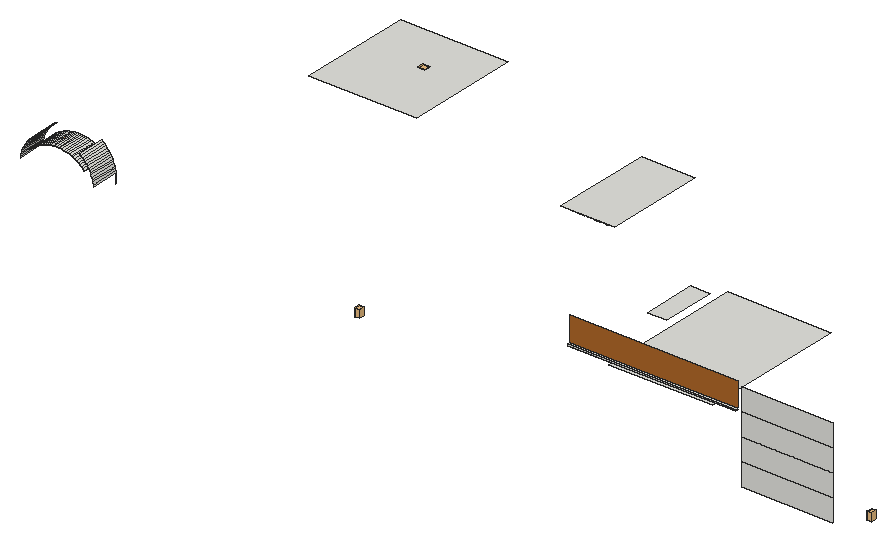
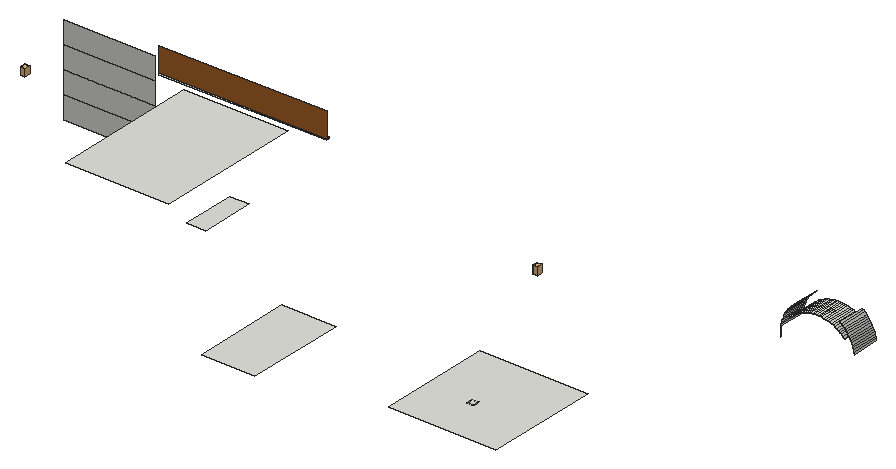
# SketchUp Ruby script. Lengths in inches.
U = 1.inch
M = Sketchup.active_model
def pt(a) = Geom::Point3d.new(a.map { |v| v * U })
def face(e, loops, mat)
  f = e.add_face(loops[0].map { |a| pt(a) })
  loops[1..].each { |l| e.add_face(l.map { |a| pt(a) }).erase! }
  f.material = f.back_material = mat if mat
  f
end
# faces: each face lists its corners as indices into pts; further lists are holes
def faces(e, pts, list, mat = nil) = list.each { |f| face(e, (f[0].is_a?(Array) ? f : [f]).map { |l| l.map { |i| pts[i] } }, mat) }
# xy, xz, yz: faces in a plane at the given z, y or x. An outline is a flat list of corners, or four numbers for a rectangle; further outlines are holes
def ring(l) = l.size == 4 ? [[l[0], l[1]], [l[2], l[1]], [l[2], l[3]], [l[0], l[3]]] : l.each_slice(2).to_a
def flat(e, list, mat, &to3) = list.each { |f| face(e, (f[0].is_a?(Array) ? f : [f]).map { |l| ring(l).map { |u, v| to3.(u, v) } }, mat) }
def xy(e, z, list, mat = nil) = flat(e, list, mat) { |x, y| [x, y, z] }
def xz(e, y, list, mat = nil) = flat(e, list, mat) { |x, z| [x, y, z] }
def yz(e, x, list, mat = nil) = flat(e, list, mat) { |y, z| [x, y, z] }
def lines(e, pts, list) = list.each { |a, b| e.add_line(pt(pts[a]), pt(pts[b])) }
# prism: a flat outline (further loops are holes) pulled along v
def prism(e, loops, v, mat = nil)
  f = face(e, loops, mat); d = Geom::Vector3d.new(v.map { |x| x * U })
  f.pushpull(f.normal.samedirection?(d) ? d.length : -d.length)
end
def box(e, o, s, mat = nil) = prism(e, [[o, [o[0] + s[0], o[1], o[2]], [o[0] + s[0], o[1] + s[1], o[2]], [o[0], o[1] + s[1], o[2]]]], [0, 0, s[2]], mat)
def at(x, y, z, deg = 0) = Geom::Transformation.translation(pt([x, y, z])) * Geom::Transformation.rotation(ORIGIN, Z_AXIS, deg.degrees)
def axes(o, x, y, z) = Geom::Transformation.new([*x, 0, *y, 0, *z, 0, *pt(o).to_a, 1])
def part(name) = M.definitions.add(name)
# library, detail: a bought-in or finely detailed component or shape, given as its bounding box
def library(name, o, s) = part(name).tap { |d| box(d.entities, o, s) }
def detail(e, o, s) = box(e.add_group.entities, o, s)
def put(e, d, t, mat = nil) = e.add_instance(d, t).tap { |i| i.material = mat if mat }
def group(e, t, mat = nil) = e.add_group.tap { |g| g.transformation = t; g.material = mat if mat }.entities
root = M.entities
M.materials.add("[Wood Bamboo]").color = [173, 103, 41]
c1 = library("Lamp Wall Outdoor 94-02",[-1.89,-4.65,-3.17],[3.78,4.65,6.35])
c2 = part("Copyright 2018, ")
xy(c2.entities,0.05,[[[19.06,0,19.06,9.82,21.3125,9.82,22.13,9.76,22.85,9.6,23.48,9.33,24,8.95,24.43,8.48,24.73,7.92,24.91,7.28,24.97,6.54,24.91,5.85,24.74,5.21,24.46,4.64,24.0625,4.14,23.58,3.73,23.03,3.4375,22.42,3.26,21.75,3.2,21.1,3.27,20.375,3.48,20.375,0],[21.62,4.3125,22.05,4.35,22.4375,4.47,22.79,4.66,23.09,4.94,23.34,5.28,23.52,5.66,23.63,6.09,23.67,6.56,23.6,7.16,23.4,7.68,23.08,8.1,22.66,8.39,22.08,8.56,21.28,8.61,20.375,8.61,20.375,4.61,20.98,4.39]],[25.77,0,27.98,4.71,25.47,9.82,26.9375,9.82,28.69,6.14,30.375,9.82,31.82,9.82,27.21,0],[[43.77,0,43.11,0.03,42.52,0.14,41.99,0.3125,41.54,0.55,41.18,0.86,40.92,1.2,40.77,1.6,40.71,2.04,40.82,2.64,41.12,3.13,41.63,3.5,42.35,3.75,41.86,4.16,41.74,4.37,41.7,4.57,41.77,4.87,41.98,5.14,42.3,5.36,42.73,5.51,42.1,5.88,41.65,6.34,41.38,6.91,41.29,7.57,41.34,8.0625,41.48,8.5,41.72,8.88,42.05,9.21,42.47,9.48,42.95,9.67,43.5,9.78,44.13,9.82,46.81,9.82,46.81,8.8125,45.49,8.8125,46.02,8.11,46.13,7.77,46.17,7.38,46.1,6.875,45.88,6.38,45.55,5.94,45.13,5.625,44.53,5.39,43.64,5.21,43.09,5.03,42.96,4.89,42.91,4.71,42.98,4.5,43.18,4.34,44.17,4.04,45.71,3.625,46.33,3.2,46.67,2.67,46.79,2.03,46.74,1.59,46.59,1.2,46.33,0.85,45.97,0.55,45.52,0.31,45.01,0.14,44.42,0.03],[43.74,1.02,44.5,1.09,45.0625,1.28,45.42,1.58,45.53,1.99,45.5,2.2,45.39,2.4,44.94,2.72,44.26,2.9375,43.41,3.01,42.82,2.94,42.34,2.73,42.03,2.42,41.93,2.03,42.04,1.59,42.38,1.28,42.95,1.09],[43.72,6.34,44.22,6.42,44.63,6.67,44.91,7.05,45,7.51,44.9,7.98,44.63,8.36,44.22,8.61,43.71,8.7,43.23,8.61,42.82,8.35,42.54,7.96,42.45,7.5,42.54,7.04,42.8125,6.67,43.22,6.42]],[180.16,0,182.36,4.71,179.85,9.82,181.32,9.82,183.07,6.14,184.75,9.82,186.2,9.82,181.59,0],[[219.8,0,219.13,0.03,218.54,0.14,218.02,0.3125,217.57,0.55,217.21,0.86,216.95,1.2,216.79,1.6,216.74,2.04,216.84,2.64,217.15,3.13,217.66,3.5,218.375,3.75,217.89,4.16,217.77,4.37,217.72,4.57,217.79,4.87,218,5.14,218.33,5.36,218.76,5.51,218.13,5.88,217.68,6.34,217.41,6.91,217.32,7.57,217.37,8.0625,217.51,8.5,217.75,8.88,218.08,9.21,218.5,9.48,218.98,9.67,219.53,9.78,220.16,9.82,222.83,9.82,222.83,8.8125,221.52,8.8125,222.05,8.11,222.16,7.77,222.2,7.38,222.125,6.875,221.91,6.38,221.58,5.94,221.16,5.625,220.5625,5.39,219.67,5.21,219.12,5.03,218.99,4.89,218.94,4.71,219.01,4.5,219.21,4.34,220.2,4.04,221.73,3.625,222.35,3.2,222.7,2.67,222.82,2.03,222.77,1.59,222.61,1.2,222.36,0.85,222,0.55,221.55,0.31,221.03,0.14,220.45,0.03],[219.77,1.02,220.53,1.09,221.09,1.28,221.44,1.58,221.5625,1.99,221.52,2.2,221.41,2.4,220.97,2.72,220.29,2.9375,219.43,3.01,218.84,2.94,218.37,2.73,218.0625,2.42,217.96,2.03,218.07,1.59,218.41,1.28,218.98,1.09],[219.75,6.34,220.25,6.42,220.66,6.67,220.93,7.05,221.02,7.51,220.93,7.98,220.66,8.36,220.24,8.61,219.74,8.7,219.25,8.61,218.85,8.35,218.57,7.96,218.48,7.5,218.57,7.04,218.84,6.67,219.25,6.42]],
  [92.62,1.6,92.62,1.87,92.89,2.17,93.07,2.48,93.22,3.3125,92.89,3.45,92.65,3.66,92.51,3.92,92.47,4.24,92.53,4.6,92.72,4.9,93.01,5.11,93.34,5.18,93.73,5.08,94.04,4.8,94.25,4.36,94.32,3.82,94.2,3.09,93.87,2.45,93.33,1.9375],[6.01,3.2,5.21,3.24,4.48,3.37,3.81,3.58,3.2,3.87,2.66,4.23,2.17,4.66,1.74,5.14,1.38,5.7,1.08,6.29,0.875,6.91,0.75,7.55,0.71,8.22,0.8,9.25,1.09,10.2,1.57,11.07,2.24,11.84,3.06,12.49,3.96,12.95,4.95,13.22,6.04,13.3125,6.83,13.26,7.68,13.11,8.5625,12.86,9.49,12.5,9.49,10.98,8.63,11.42,7.78,11.72,6.9375,11.91,6.11,11.97,5.29,11.9,4.55,11.7,3.89,11.37,3.29,10.9,2.8,10.33,2.45,9.7,2.24,8.99,2.17,8.22,2.24,7.44,2.45,6.74,2.79,6.11,3.27,5.55,3.86,5.09,4.53,4.76,5.27,4.57,6.09,4.5,6.98,4.57,7.87,4.78,8.74,5.12,9.6,5.6,9.6,4.05,8.79,3.68,7.92,3.41,6.99,3.25],[[14.21,3.2,13.51,3.26,12.87,3.4375,12.29,3.73,11.77,4.14,11.34,4.65,11.03,5.21,10.85,5.82,10.78,6.5,10.85,7.1875,11.03,7.81,11.34,8.375,11.78,8.88,12.31,9.3,12.9,9.59,13.55,9.77,14.27,9.83,14.98,9.77,15.63,9.59,16.21,9.29,16.73,8.87,17.16,8.36,17.47,7.79,17.66,7.16,17.72,6.47,17.66,5.79,17.47,5.18,17.16,4.625,16.72,4.13,16.19,3.72,15.6,3.43,14.9375,3.26],[14.25,4.4,14.71,4.44,15.12,4.55,15.48,4.74,15.81,5,16.07,5.32,16.26,5.68,16.37,6.08,16.41,6.53,16.37,6.97,16.25,7.375,16.06,7.74,15.78,8.0625,15.45,8.33,15.07,8.52,14.65,8.63,14.2,8.67,13.76,8.63,13.36,8.52,13,8.33,12.68,8.0625,12.42,7.74,12.23,7.37,12.12,6.97,12.08,6.52,12.12,6.07,12.24,5.67,12.43,5.31,12.69,4.99,13.02,4.73,13.39,4.55,13.8,4.44]],[57.3125,3.2,56.51,3.33,55.84,3.72,55.54,4.07,55.34,4.58,55.26,5.77,55.26,8.66,54.13,8.66,54.13,8.78,56.54,11.16,56.54,9.82,58.6,9.82,58.6,8.66,56.54,8.66,56.54,5.48,56.6,4.99,56.78,4.64,57.06,4.43,57.47,4.36,58.18,4.48,58.93,4.82,58.93,3.62,58.16,3.31],[[88.3125,3.2,87.67,3.25,87.08,3.41,86.54,3.66,86.06,4.02,85.66,4.45,85.37,4.93,85.2,5.46,85.14,6.04,85.23,6.75,85.49,7.37,85.93,7.91,86.54,8.36,86,8.86,85.64,9.37,85.4375,9.91,85.37,10.54,85.43,11.1,85.59,11.61,85.86,12.08,86.24,12.51,86.7,12.86,87.21,13.11,87.76,13.26,88.37,13.3125,88.96,13.26,89.51,13.11,90.01,12.86,90.46,12.51,90.83,12.09,91.09,11.62,91.25,11.1,91.31,10.54,91.23,9.91,91,9.33,90.62,8.82,90.08,8.36,90.68,7.91,91.11,7.38,91.36,6.75,91.45,6.02,91.39,5.4375,91.23,4.91,90.95,4.43,90.56,4,90.08,3.65,89.55,3.4,88.96,3.25],[88.33,4.54,89,4.64,89.54,4.94,89.9,5.39,90.02,5.96,90.02,6.11,89.9,6.72,89.54,7.21,88.98,7.53,88.28,7.64,87.6,7.53,87.05,7.21,86.69,6.71,86.57,6.09,86.69,5.47,87.06,4.98,87.62,4.65],[88.35,9.02,88.95,9.125,89.45,9.45,89.79,9.93,89.9,10.49,89.79,11.08,89.46,11.55,88.96,11.87,88.34,11.97,87.72,11.87,87.22,11.5625,86.89,11.09,86.78,10.51,86.89,9.9375,87.24,9.46,87.75,9.13]],
  [[113.29,3.2,112.92,3.24,112.64,3.36,112.43,3.57,112.32,3.85,111.9,3.57,111.47,3.375,111.03,3.26,110.57,3.22,109.95,3.33,109.44,3.66,109.1,4.17,108.99,4.79,109.1,5.375,109.43,5.89,109.97,6.32,110.6875,6.66,112.33,7.22,112.33,7.57,112.26,8.08,112.04,8.45,111.67,8.67,111.16,8.74,110.64,8.67,110.12,8.47,109.61,8.13,109.11,7.65,109.11,9.06,109.53,9.45,110.02,9.72,110.6,9.89,111.27,9.94,111.77,9.91,112.21,9.81,112.61,9.63,112.95,9.39,113.34,8.92,113.55,8.34,113.6,7.22,113.6,4.46,113.65,4.21,113.82,4.13,114.12,4.21,114.55,4.47,114.55,3.6875,113.85,3.3],[111.19,4.1,111.79,4.22,112.33,4.6,112.33,6.53,111.47,6.2,110.91,5.9375,110.54,5.67,110.34,5.375,110.27,5.01,110.33,4.64,110.53,4.35,110.82,4.16]],[121.02,3.2,120.43,3.28,119.88,3.51,119.43,3.87,119.1,4.34,118.9,5.04,118.83,6.09,118.83,9.82,120.12,9.82,120.12,6.11,120.19,5.24,120.41,4.68,120.82,4.38,121.44,4.28,121.88,4.33,122.29,4.5,122.66,4.78,123,5.17,123,9.82,124.29,9.82,124.29,3.3125,123,3.3125,123,4.15,122.5625,3.75,122.07,3.45,121.54,3.26],[[156.36,3.2,155.99,3.24,155.7,3.36,155.5,3.57,155.39,3.85,154.97,3.57,154.54,3.375,154.1,3.26,153.64,3.22,153.02,3.33,152.51,3.66,152.17,4.17,152.06,4.79,152.17,5.375,152.5,5.89,153.03,6.32,153.75,6.66,155.4,7.22,155.4,7.57,155.33,8.08,155.11,8.45,154.74,8.67,154.23,8.74,153.7,8.67,153.1875,8.47,152.68,8.13,152.18,7.65,152.18,9.06,152.59,9.45,153.09,9.72,153.67,9.89,154.33,9.94,154.83,9.91,155.28,9.81,155.68,9.63,156.02,9.39,156.4,8.92,156.62,8.34,156.66,7.22,156.66,4.46,156.72,4.21,156.89,4.13,157.1875,4.21,157.62,4.47,157.62,3.6875,156.92,3.3],[154.26,4.1,154.85,4.22,155.4,4.6,155.4,6.53,154.54,6.2,153.98,5.9375,153.61,5.67,153.4,5.375,153.34,5.01,153.4,4.64,153.59,4.35,153.89,4.16]],[161.74,3.2,161.01,3.26,160.37,3.43,159.8,3.71,159.3,4.11,158.91,4.6,158.62,5.16,158.45,5.81,158.4,6.53,158.45,7.26,158.62,7.92,158.89,8.5,159.28,9,159.76,9.41,160.3,9.71,160.92,9.88,161.6,9.94,162.51,9.85,163.49,9.49,163.49,8.12,162.55,8.59,161.68,8.74,161.27,8.7,160.89,8.59,160.55,8.4,160.25,8.13,160.01,7.8,159.84,7.4375,159.73,7.02,159.7,6.57,159.73,6.1,159.85,5.68,160.04,5.31,160.3,4.99,160.63,4.73,161.01,4.55,161.44,4.4375,161.93,4.4,162.73,4.51,163.63,4.83,163.63,3.5625,162.67,3.29],[[178.37,3.2,178,3.24,177.71,3.36,177.51,3.57,177.39,3.85,176.98,3.57,176.55,3.375,176.1,3.26,175.65,3.22,175.02,3.33,174.52,3.66,174.18,4.17,174.0625,4.79,174.17,5.375,174.51,5.89,175.04,6.32,175.76,6.66,177.41,7.22,177.41,7.57,177.33,8.08,177.11,8.45,176.75,8.67,176.23,8.74,175.71,8.67,175.19,8.47,174.6875,8.13,174.18,7.65,174.18,9.06,174.6,9.45,175.1,9.72,175.68,9.89,176.34,9.94,176.84,9.91,177.29,9.81,177.68,9.63,178.03,9.39,178.41,8.92,178.625,8.34,178.67,7.22,178.67,4.46,178.73,4.21,178.9,4.13,179.2,4.21,179.625,4.47,179.625,3.6875,178.92,3.3],[176.27,4.1,176.86,4.22,177.41,4.6,177.41,6.53,176.54,6.2,175.98,5.9375,175.61,5.67,175.41,5.375,175.34,5.01,175.41,4.64,175.6,4.35,175.9,4.16]],
  [210.76,3.2,209.73,3.33,208.59,3.78,208.59,5.17,209.71,4.55,210.23,4.37,210.66,4.3125,211.04,4.36,211.36,4.51,211.57,4.73,211.65,4.98,211.6,5.24,211.46,5.45,210.65,5.99,209.62,6.64,209.02,7.18,208.73,7.69,208.64,8.25,208.67,8.6,208.78,8.93,208.96,9.22,209.22,9.47,209.89,9.83,210.72,9.94,211.6875,9.81,212.68,9.41,212.68,8.13,211.64,8.65,210.81,8.83,210.47,8.79,210.2,8.67,210.03,8.48,209.97,8.25,210.02,8.03,210.18,7.82,210.91,7.32,211.37,7.06,212.08,6.59,212.59,6.09,212.89,5.57,213,5.02,212.96,4.64,212.84,4.3,212.64,3.99,212.37,3.71,212.04,3.49,211.66,3.33],[[73.82,3.22,73.14,3.3,72.53,3.56,71.99,3.99,71.52,4.59,71.14,5.34,70.87,6.2,70.7,7.17,70.65,8.25,70.71,9.32,70.875,10.29,71.16,11.15,71.55,11.9,72.03,12.52,72.58,12.96,73.2,13.23,73.88,13.3125,74.53,13.23,75.12,12.96,75.65,12.51,76.125,11.89,76.51,11.13,76.79,10.27,76.96,9.32,77.01,8.28,76.96,7.2,76.79,6.24,76.51,5.38,76.125,4.62,75.65,4.01,75.11,3.57,74.5,3.3],[73.81,4.52,74.2,4.58,74.54,4.77,74.84,5.08,75.1,5.51,75.31,6.06,75.46,6.6875,75.58,8.22,75.46,9.76,75.32,10.4,75.12,10.95,74.87,11.4,74.59,11.72,74.26,11.91,73.89,11.97,73.82,11.97,73.4375,11.91,73.09,11.72,72.79,11.41,72.53,10.97,72.32,10.43,72.18,9.79,72.06,8.26,72.17,6.7,72.32,6.06,72.52,5.51,72.78,5.08,73.08,4.77,73.42,4.58]],[[204.86,3.22,203.89,3.33,203.125,3.66,202.53,4.18,202.06,4.86,201.76,5.67,201.66,6.6,201.71,7.31,201.87,7.95,202.13,8.51,202.5,9.01,202.95,9.42,203.47,9.71,204.05,9.89,204.6875,9.94,205.3,9.89,205.85,9.72,206.33,9.43,206.75,9.04,207.09,8.55,207.33,7.98,207.47,7.34,207.52,6.61,207.52,6.45,202.95,6.45,203.13,5.61,203.32,5.27,203.57,4.97,203.88,4.73,204.23,4.55,205.06,4.42,205.68,4.47,206.28,4.61,206.86,4.86,207.41,5.21,207.41,3.95,206.82,3.61,206.23,3.39,205.6,3.26],[202.98,7.22,206.25,7.22,206.11,7.9,205.79,8.41,205.31,8.72,204.6875,8.83,204.06,8.72,203.55,8.41,203.1875,7.9]],[32.81,3.3125,32.81,9.82,34.1,9.82,34.1,8.33,34.17,8.4375,34.64,9.1,35.1,9.57,35.57,9.85,36.04,9.94,36.4,9.9,36.78,9.76,37.55,9.21,36.875,8.08,36.23,8.55,35.63,8.71,35.33,8.68,35.05,8.57,34.55,8.12,34.21,7.47,34.1,6.71,34.1,3.3125],[38.48,3.3125,39.77,9.82],
  [47.77,3.3125,47.77,13.1875,49.06,13.1875,49.06,8.96,49.49,9.39,49.96,9.7,50.49,9.88,51.06,9.94,51.68,9.86,52.23,9.62,52.68,9.23,52.99,8.72,53.18,8.01,53.24,7.02,53.24,3.3125,51.96,3.3125,51.96,7.34,51.87,7.98,51.61,8.48,51.2,8.81,50.6875,8.92,50.27,8.86,49.89,8.7,49.49,8.41,49.06,7.97,49.06,3.3125],[63.46,3.3125,63.46,3.41,64.06,4.11,66.27,7.04,66.95,8.09,67.35,8.86,67.53,9.47,67.6,10.07,67.48,10.82,67.125,11.41,66.57,11.79,65.87,11.92,65.28,11.83,64.7,11.57,64.15,11.14,63.66,10.58,63.66,12.375,64.24,12.79,64.83,13.08,65.43,13.26,66.04,13.3125,66.65,13.26,67.21,13.1,67.72,12.83,68.17,12.45,68.53,11.99,68.79,11.47,68.95,10.9,69,10.26,68.95,9.65,68.8,8.99,68.51,8.27,68.06,7.4375,67.34,6.4,66.26,5.04,65.95,4.68,69.71,4.68,69.71,3.3125],[80.37,3.3125,81.78,13.1875],[100.21,3.3125,100.21,13.1875,101.625,13.1875,101.625,8.67,105.78,13.1875,107.55,13.1875,103.27,8.5,108.6,3.3125,106.67,3.3125,101.625,8.19,101.625,3.3125],[115.72,3.3125,117,13.1875],
  [126.04,3.3125,126.04,9.82,127.33,9.82,127.33,8.96,127.82,9.39,128.3,9.7,128.78,9.88,129.25,9.94,129.83,9.87,130.35,9.65,130.79,9.28,131.17,8.77,131.6875,9.29,132.22,9.66,132.77,9.88,133.32,9.96,133.77,9.91,134.18,9.78,134.55,9.57,134.88,9.27,135.15,8.875,135.34,8.39,135.45,7.82,135.49,7.15,135.49,3.3125,134.2,3.3125,134.2,7.17,134.12,7.88,133.87,8.41,133.47,8.73,132.92,8.84,132.53,8.79,132.15,8.64,131.78,8.39,131.43,8.04,131.43,3.3125,130.13,3.3125,130.13,6.93,130.0625,7.85,129.84,8.44,129.67,8.63,129.45,8.76,128.83,8.87,128.45,8.82,128.1,8.6875,127.74,8.43,127.33,8.04,127.33,3.3125],[141.43,3.3125,141.43,13.1875,142.77,13.1875,146.05,9.13,149.31,13.1875,150.63,13.1875,150.63,3.3125,149.21,3.3125,149.21,11,146.17,7.18,145.91,7.18,142.84,11,142.84,3.3125],[165.29,3.3125,165.29,13.1875,166.7,13.1875,166.7,8.67,170.86,13.1875,172.62,13.1875,168.34,8.5,173.67,3.3125,171.75,3.3125,166.7,8.19,166.7,3.3125],[214.51,3.3125,215.8,9.82],[223.8,3.3125,223.8,9.82,225.12,9.82,225.12,8.99,225.5625,9.41,226.04,9.7,226.54,9.88,227.07,9.94,227.66,9.86,228.2,9.63,228.67,9.26,229,8.77,229.2,8.06,229.27,7.03,229.27,3.3125,227.99,3.3125,227.99,7.02,227.91,7.87,227.68,8.44,227.28,8.76,226.66,8.87,226.23,8.8125,225.82,8.64,225.45,8.36,225.12,7.96,225.12,3.3125],
  [[191.3125,3.33,191.3125,13.1875,194.64,13.1875,195.6,13.15,196.45,13.04,197.19,12.85,197.83,12.58,198.39,12.25,198.88,11.84,199.32,11.36,199.7,10.81,200,10.21,200.22,9.58,200.35,8.93,200.39,8.25,200.29,7.28,200.01,6.35,199.54,5.5,198.92,4.76,198.14,4.14,197.24,3.7,196.22,3.4,194.4375,3.33],[192.73,4.59,194.54,4.59,195.48,4.62,196.18,4.73,197.16,5.1,197.88,5.65,198.34,6.21,198.66,6.85,198.86,7.55,198.93,8.33,198.86,9.08,198.66,9.77,198.32,10.38,197.85,10.92,197.43,11.26,196.94,11.53,195.97,11.85,194.49,11.93,192.73,11.93]],[39.12,11.03,38.84,11.09,38.59,11.26,38.42,11.51,38.37,11.8,38.42,12.08,38.59,12.32,38.84,12.49,39.12,12.55,39.41,12.5,39.66,12.33,39.83,12.09,39.89,11.8,39.83,11.51,39.66,11.26,39.41,11.09],[215.14,11.03,214.87,11.09,214.62,11.26,214.45,11.51,214.4,11.8,214.45,12.08,214.62,12.32,214.87,12.49,215.14,12.55,215.44,12.5,215.6875,12.33,215.86,12.09,215.92,11.8,215.86,11.51,215.6875,11.26,215.44,11.09]])
c3 = library("Spot Light",[-8.21,-8.21,-2.75],[16.42,16.42,2.75])
c4 = library("Omni Light",[-12,-12,-12],[24,24,24])
xy(root,320.98,[[834.07,1080.1875,878.82,1163.875]])
xy(root,326.83,[[973.0625,997.25,988.8125,1041.93]])
xy(root,334.79,[[1005.21,916.1875,1091.46,1039.625]])
xy(root,339.08,[[973.0625,913.52,1112.75,916.1875]])
xy(root,340.08,[[973.0625,913.52,1112.75,916.1875]])
xy(root,342.64,[[586.375,893.4375,587,916.1875]])
xy(root,344.51,[[624.25,1080.1875,714.02,1175.3125]])
xz(root,913.52,[[973.0625,339.08,1112.75,340.08]])
xz(root,916.1875,[[594.375,325.32,594.46,326.15,594.375,326.72],[594.46,326.15,594.55,326.93,594.63,328.54,594.64,330.16,594.56,331.77,594.39,333.38,594.375,333.47,594.375,326.72]])
xz(root,916.1875,[[973.0625,340.08,1112.75,360.64]],"[Wood Bamboo]")
xz(root,919.75,[[1112.75,279.91,1189.1875,298.51],[1112.75,298.51,1189.1875,317.11],[1112.75,317.11,1189.1875,335.71],[1112.75,335.71,1189.1875,354.31]])
p = [[533.44,916.1875,335.09],[533.1875,916.1875,333.49],[533.1875,893.4375,333.49],[533.44,893.4375,335.09],[594.375,916.1875,333.47],[594.14,916.1875,334.98],
  [594.14,893.4375,334.98],[594.375,893.4375,333.47],[593.81,916.1875,336.56],[593.81,893.4375,336.56],[533.78,916.1875,336.67],[533.78,893.4375,336.67],
  [593.39,916.1875,338.12],[593.39,893.4375,338.12],[534.2,916.1875,338.23],[534.2,893.4375,338.23],[592.89,916.1875,339.66],[592.89,893.4375,339.66],
  [534.7,916.1875,339.76],[534.7,893.4375,339.76],[592.32,916.1875,341.17],[592.32,893.4375,341.17],[535.29,916.1875,341.27],[535.29,893.4375,341.27],
  [591.66,916.1875,342.65],[591.66,893.4375,342.65],[535.95,916.1875,342.74],[535.95,893.4375,342.74],[541.1875,916.1875,342.21],[541.625,916.1875,342.7],
  [541.625,893.4375,342.7],[541.1875,893.4375,342.21],[585.26,916.1875,343.76],[586.375,916.1875,342.64],[586.375,893.4375,342.64],[585.26,893.4375,343.76],
  [590.93,916.1875,344.09],[590.93,893.4375,344.09],[536.68,916.1875,344.18],[536.68,893.4375,344.18],[542.77,916.1875,343.84],[542.77,893.4375,343.84],
  [543.97,916.1875,344.92],[543.97,893.4375,344.92],[584.0625,916.1875,344.84],[584.0625,893.4375,344.84],[590.125,916.1875,345.49],[590.125,893.4375,345.49],
  [537.49,916.1875,345.58],[537.49,893.4375,345.58],[582.81,916.1875,345.86],[582.81,893.4375,345.86],[545.23,916.1875,345.93],[545.23,893.4375,345.93],
  [589.25,916.1875,346.84],[589.25,893.4375,346.84],[538.375,916.1875,346.93],[538.375,893.4375,346.93],[546.54,916.1875,346.88],[546.54,893.4375,346.88],
  [581.5,916.1875,346.82],[581.5,893.4375,346.82],[580.15,916.1875,347.7],[580.15,893.4375,347.7],[588.3,916.1875,348.15],[588.3,893.4375,348.15],
  [539.33,916.1875,348.24],[539.33,893.4375,348.24],[547.9,916.1875,347.76],[547.9,893.4375,347.76],[578.75,916.1875,348.51],[578.75,893.4375,348.51],
  [549.3,916.1875,348.5625],[549.3,893.4375,348.5625],[540.35,916.1875,349.49],[540.35,893.4375,349.49],[587.29,916.1875,349.41],[587.29,893.4375,349.41],
  [577.3125,916.1875,349.24],[577.3125,893.4375,349.24],[550.74,916.1875,349.29],[550.74,893.4375,349.29],[575.84,916.1875,349.9],[575.84,893.4375,349.9],
  [552.22,916.1875,349.95],[552.22,893.4375,349.95],[586.21,916.1875,350.61],[586.21,893.4375,350.61],[541.43,916.1875,350.69],[541.43,893.4375,350.69],
  [553.73,916.1875,350.52],[553.73,893.4375,350.52],[574.33,916.1875,350.49],[574.33,893.4375,350.49],[555.26,916.1875,351.02],[555.26,893.4375,351.02],
  [572.8,916.1875,350.99],[572.8,893.4375,350.99],[585.07,916.1875,351.76],[585.07,893.4375,351.76],[542.58,916.1875,351.83],[542.58,893.4375,351.83],
  [556.82,916.1875,351.43],[556.82,893.4375,351.43],[571.24,916.1875,351.41],[571.24,893.4375,351.41],[558.41,916.1875,351.77],[558.41,893.4375,351.77],
  [569.66,916.1875,351.75],[569.66,893.4375,351.75],[568.06,916.1875,352],[568.06,893.4375,352],[543.78,916.1875,352.91],[543.78,893.4375,352.91],
  [560,916.1875,352.02],[560,893.4375,352.02],[583.87,916.1875,352.84],[583.87,893.4375,352.84],[561.61,916.1875,352.18],[561.61,893.4375,352.18],
  [566.45,916.1875,352.18],[566.45,893.4375,352.18],[563.22,916.1875,352.27],[563.22,893.4375,352.27],[564.84,916.1875,352.26],[564.84,893.4375,352.26],
  [582.61,916.1875,353.86],[582.61,893.4375,353.86],[545.04,916.1875,353.93],[545.04,893.4375,353.93]]
faces(root,p,[[0,1,2,3],[4,5,6,7],[5,8,9,6],[10,0,3,11],[8,12,13,9],[14,10,11,15],[12,16,17,13],[18,14,15,19],
  [16,20,21,17],[22,18,19,23],[20,24,25,21],[26,22,23,27],[28,29,30,31],[32,33,34,35],[24,36,37,25],[38,26,27,39],
  [29,40,41,30],[40,42,43,41],[44,32,35,45],[36,46,47,37],[48,38,39,49],[50,44,45,51],[42,52,53,43],[46,54,55,47],
  [56,48,49,57],[52,58,59,53],[60,50,51,61],[62,60,61,63],[54,64,65,55],[66,56,57,67],[58,68,69,59],[70,62,63,71],
  [68,72,73,69],[74,66,67,75],[64,76,77,65],[78,70,71,79],[72,80,81,73],[82,78,79,83],[80,84,85,81],[76,86,87,77],
  [88,74,75,89],[84,90,91,85],[92,82,83,93],[90,94,95,91],[96,92,93,97],[86,98,99,87],[100,88,89,101],[94,102,103,95],
  [104,96,97,105],[102,106,107,103],[108,104,105,109],[110,108,109,111],[112,100,101,113],[106,114,115,107],[98,116,117,99],[114,118,119,115],
  [120,110,111,121],[118,122,123,119],[124,120,121,125],[122,124,125,123],[116,126,127,117],[128,112,113,129]])
put(root,c1,at(1226.05,916.1875,301.26))
put(root,c1,at(799.21,916.1875,303.08))
put(root,c2,axes([872.05,1084.14,319.47],[-0.13928,0,0],[0,-0.1494,0],[0,0,0.93236]))
put(root,c3,axes([675.26,1136.06,344.51],[0.32,0,0],[0,0.32,0],[0,0,0.32]))
put(root,c4,axes([560.86,905.86,350.2],[0.14094,0,0],[0,0.14094,0],[0,0,0.14094]))
